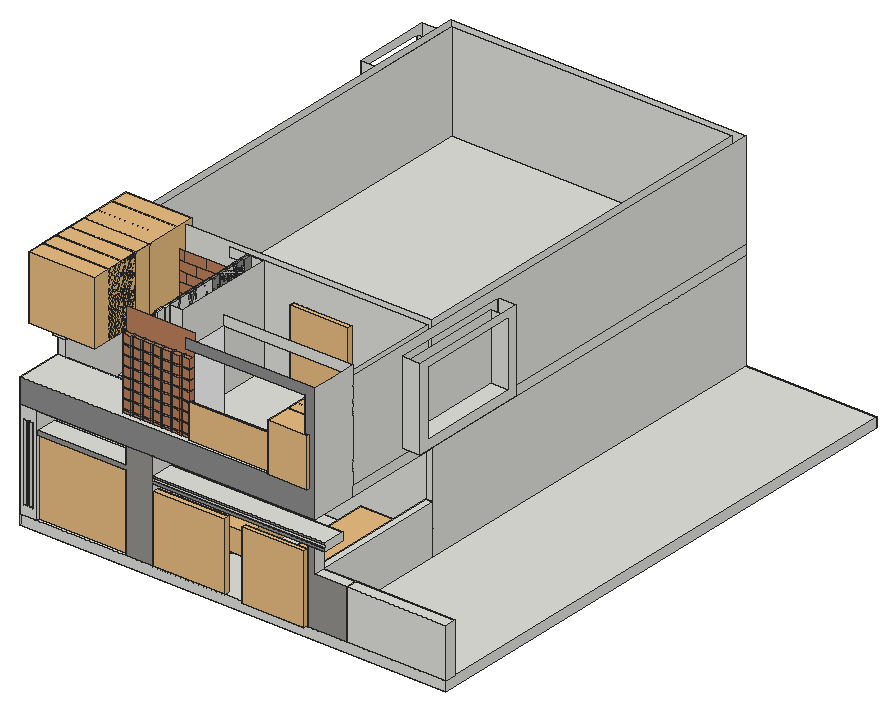
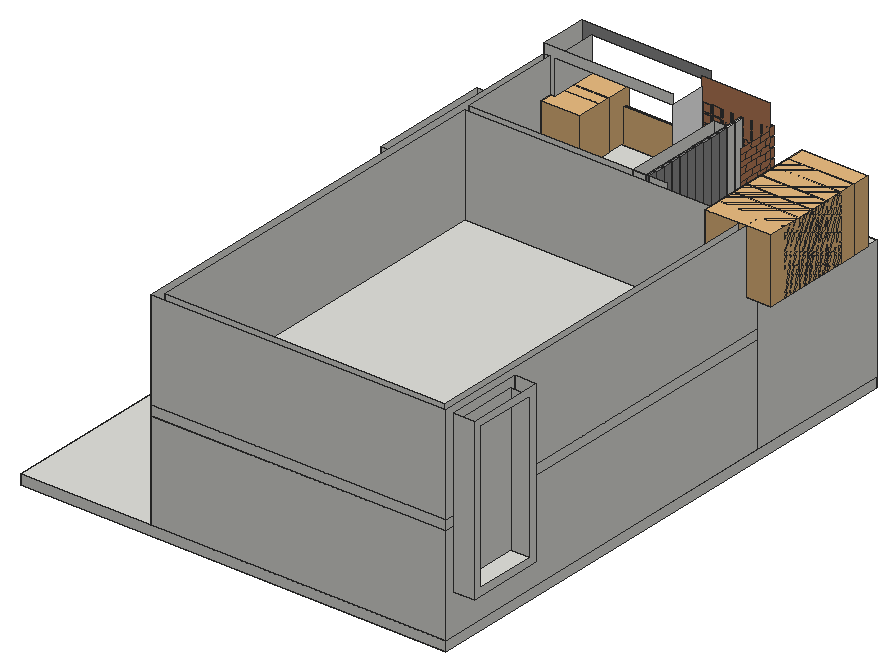
# SketchUp Ruby script. Lengths in inches.
U = 1.inch
M = Sketchup.active_model
def pt(a) = Geom::Point3d.new(a.map { |v| v * U })
def face(e, loops, mat)
  f = e.add_face(loops[0].map { |a| pt(a) })
  loops[1..].each { |l| e.add_face(l.map { |a| pt(a) }).erase! }
  f.material = f.back_material = mat if mat
  f
end
# faces: each face lists its corners as indices into pts; further lists are holes
def faces(e, pts, list, mat = nil) = list.each { |f| face(e, (f[0].is_a?(Array) ? f : [f]).map { |l| l.map { |i| pts[i] } }, mat) }
# xy, xz, yz: faces in a plane at the given z, y or x. An outline is a flat list of corners, or four numbers for a rectangle; further outlines are holes
def ring(l) = l.size == 4 ? [[l[0], l[1]], [l[2], l[1]], [l[2], l[3]], [l[0], l[3]]] : l.each_slice(2).to_a
def flat(e, list, mat, &to3) = list.each { |f| face(e, (f[0].is_a?(Array) ? f : [f]).map { |l| ring(l).map { |u, v| to3.(u, v) } }, mat) }
def xy(e, z, list, mat = nil) = flat(e, list, mat) { |x, y| [x, y, z] }
def xz(e, y, list, mat = nil) = flat(e, list, mat) { |x, z| [x, y, z] }
def yz(e, x, list, mat = nil) = flat(e, list, mat) { |y, z| [x, y, z] }
def lines(e, pts, list) = list.each { |a, b| e.add_line(pt(pts[a]), pt(pts[b])) }
# prism: a flat outline (further loops are holes) pulled along v
def prism(e, loops, v, mat = nil)
  f = face(e, loops, mat); d = Geom::Vector3d.new(v.map { |x| x * U })
  f.pushpull(f.normal.samedirection?(d) ? d.length : -d.length)
end
def box(e, o, s, mat = nil) = prism(e, [[o, [o[0] + s[0], o[1], o[2]], [o[0] + s[0], o[1] + s[1], o[2]], [o[0], o[1] + s[1], o[2]]]], [0, 0, s[2]], mat)
def at(x, y, z, deg = 0) = Geom::Transformation.translation(pt([x, y, z])) * Geom::Transformation.rotation(ORIGIN, Z_AXIS, deg.degrees)
def axes(o, x, y, z) = Geom::Transformation.new([*x, 0, *y, 0, *z, 0, *pt(o).to_a, 1])
def part(name) = M.definitions.add(name)
# library, detail: a bought-in or finely detailed component or shape, given as its bounding box
def library(name, o, s) = part(name).tap { |d| box(d.entities, o, s) }
def detail(e, o, s) = box(e.add_group.entities, o, s)
def put(e, d, t, mat = nil) = e.add_instance(d, t).tap { |i| i.material = mat if mat }
def group(e, t, mat = nil) = e.add_group.tap { |g| g.transformation = t; g.material = mat if mat }.entities
root = M.entities
M.materials.add("[Color M00]").color = [255, 255, 255]
M.materials.add("[Color M04]").color = [142, 142, 142]
M.materials.add("[Granite Light Gray]").color = [149, 148, 144]
M.materials.add("[Wood Veneer 02]").color = [190, 128, 91]
c1 = library("Untitled",[-140.43,-165.12,-406.46],[82.02,2.41,46.46])
c2 = library("Double metal gate",[0,0,0],[87.31,5.6,111.9])
c3 = library("mercy",[0,0.0625,0.17],[86.93,197.26,61.05])
c4 = library("skp127A",[-867.34,-144.26,-31.81],[70.33,146.61,36.4])
c5 = library("ske10",[-0.02,0,-0.02],[0.61,0.21,0.61])
c6 = part("Group\#44")
put(c6.entities,c5,axes([0,3814.77,792.79],[0,-1379.55262,0],[1876.19156,0,0],[0,0,-1379.55262]))
put(c6.entities,c5,axes([8.16,779.46,780.08],[0,-1356.35677,0],[1356.35677,0,0],[0,0,-1356.35677]))
c7 = part("ske69")
put(c7.entities,c4,axes([28413.25,5172.05,1237.79],[36.65,0,0],[0,36.65,0],[0,0,36.65]))
put(c7.entities,c6,at(-3177.4,833.5,-0.89))
put(c7.entities,c6,axes([-1005.07,821.63,0],[-1,0,0],[0,1,0],[0,0,1]))
c8 = part("Untitled\#1")
put(c8.entities,c7,axes([477.34,-958.1,-17.4375],[0.1036,0,0],[0,0.1036,0],[0,0,0.1036]))
c9 = part("Group\#156")
prism(c9.entities,[[[0,0,0],[0,10.0625,0],[0,10.0625,0.9],[0,10.0625,12],[0,10.0625,12.9],[0,10.0625,24.9],[0,10.0625,36.9],[0,10.0625,48.9],[0,10.0625,60.9],[0,10.0625,72.9],[0,10.0625,84.9],[0,10.0625,96.9],[0,10.0625,108.9],[0,10.0625,120.9],[0,10.0625,131.875],[0,0,131.875]]],[-3.5625,0,0])
c10 = part("Group\#155")
box(c10.entities,[0,0,0],[10,10,5.4375],"[Color M00]")
c11 = library("glass door",[0,0,0],[6.2,71.19,86.61])
c12 = library("Wagner Glass Railing",[9.08,102.375,1.53],[2.51,145.5,42.05])
c13 = library("KentiaPalm",[-22.86,-14.31,0],[47.49,43.96,59.125])
c14 = library("Round Planter with Plant",[-35.48,-39.77,0],[80.62,63.55,77.875])
xy(root,0,[[34.0625,4.36,54.1875,61.36],[162.77,4.36,196.52,30.99],[385.0625,4.43,385.0625,61.36,394.0625,61.36,394.0625,17.84,433,17.84,433,4.43],[433,4.43,554.0625,17.84],[34.0625,61.36,44.1875,184.55],
  [[44.1875,61.36,185.125,61.36,185.125,184.55,394.0625,184.55,394.0625,661.36,34.0625,661.36,34.0625,184.55,44.1875,184.55],[43.0625,193.55,385.0625,652.36]],[185.125,61.36,385.0625,70.36],[185.125,70.36,385.0625,184.55],[43.0625,193.55,385.0625,652.36]])
xy(root,11.32,[[45.66,4.36,49.72,7.36]])
xy(root,11.5,[[38.65,4.36,42.71,7.36]])
xy(root,12,[[44.1875,61.36,171.15,68.43]])
xy(root,24,[[44.1875,68.43,171.15,80.43]])
xy(root,36,[[44.1875,80.43,171.15,92.43]])
xy(root,48,[[44.1875,92.43,171.15,104.43]])
xy(root,49.1875,[[7.8125,556.61,34.0625,650.86]])
xy(root,58.14,[[7.8125,565.56,31.8125,641.91]])
xy(root,60,[[44.1875,104.43,171.15,116.43]])
xy(root,60.375,[[394.0625,4.43,433,17.84],[433,4.43,554.0625,17.84],[385.0625,17.84,394.0625,184.55]])
xy(root,72,[[44.1875,116.43,171.15,128.43]])
xy(root,84,[[44.1875,128.43,171.15,140.43]])
xy(root,89.1875,[[385.0625,4.43,394.0625,17.84]])
xy(root,89.38,[[196.52,4.36,406.2,30.99]])
xy(root,92.78,[[196.33,4.36,406.2,5.86]])
xy(root,93.625,[[54.14,4.36,162.77,30.99]])
xy(root,96,[[44.1875,140.43,171.15,152.43]])
xy(root,96.47,[[196.33,4.36,406.2,5.86]])
xy(root,98.53,[[54.14,4.36,162.77,30.99]])
xy(root,99.1875,[[196.52,4.36,406.2,30.99]])
xy(root,105.3125,[[38.65,4.36,42.71,7.36]])
xy(root,105.57,[[45.66,4.36,49.72,7.36]])
xy(root,108,[[44.1875,152.43,171.15,164.43]])
xy(root,120,[[54.1875,4.36,54.1875,61.36,394.0625,61.36,394.0625,4.36,196.52,4.36,196.52,30.99,162.77,30.99,162.77,4.36],[171.15,61.36,185.125,184.55],[185.125,61.36,394.0625,184.55],[44.1875,164.43,171.15,184.55],[[34.0625,184.55,394.0625,661.36],[43.0625,193.55,385.0625,652.36]]])
xy(root,132,[[187.02,61.36,394.0625,61.36,394.0625,61.62,387.09,61.62,387.09,184.55,187.02,184.55],[387.09,61.62,394.0625,184.55],[43.0625,193.55,385.0625,652.36]])
xy(root,140.375,[[394.0625,137.15,416.125,283.4]])
xy(root,150.125,[[34.0625,4.36,381.58,4.36,381.58,61.36,236.46,61.36,236.46,17.17,153.47,17.17,153.47,61.36,34.0625,61.36],[153.47,17.17,171.15,61.36],[171.15,17.17,236.46,61.36]])
xy(root,151.78,[[394.0625,149.62,416.125,272.62]])
xy(root,171.9375,[[31.4375,56.86,31.4375,184.55,34.0625,184.55,34.0625,61.36,44.1875,61.36,44.1875,184.55,47.125,184.55,47.125,56.86],[34.0625,61.36,44.1875,184.55]])
xy(root,175.625,[[31.4375,56.86,47.125,184.55]])
xz(root,4.36,[[[34.0625,0,54.1875,0,54.1875,93.625,54.14,93.625,54.14,98.53,54.1875,98.53,54.1875,120,34.0625,120],[45.66,11.32,49.72,105.57],[38.65,11.5,42.71,105.3125]],[54.14,93.625,54.1875,98.53]])
xz(root,4.36,[[34.0625,120,394.0625,120,394.0625,264,236.46,264,236.46,252,381.58,252,381.58,150.125,34.0625,150.125]],"[Color M04]")
xz(root,4.36,[[162.77,0,196.52,0,196.52,89.38,406.2,89.38,406.2,92.78,196.33,92.78,196.33,96.47,406.2,96.47,406.2,99.1875,196.52,99.1875,196.52,120,162.77,120,162.77,98.53,54.1875,98.53,54.1875,93.625,162.77,93.625]],"[Granite Light Gray]")
xz(root,4.43,[[433,0,554.0625,60.375]])
xz(root,4.43,[[385.0625,0,433,0,433,60.375,394.0625,60.375,394.0625,89.1875,385.0625,89.1875]],"[Granite Light Gray]")
xz(root,5.86,[[196.33,92.78,406.2,96.47]])
xz(root,7.36,[[45.66,11.32,49.72,105.57],[38.65,11.5,42.71,105.3125]])
xz(root,17.17,[[153.47,150.125,236.46,264]],"[Wood Veneer 02]")
xz(root,17.84,[[394.0625,0,433,60.375],[433,0,554.0625,60.375],[385.0625,60.375,394.0625,89.1875]])
xz(root,30.99,[[162.77,0,162.77,93.625,54.14,93.625,54.14,98.53,162.77,98.53,162.77,120,196.52,120,196.52,99.1875,406.2,99.1875,406.2,89.38,196.52,89.38,196.52,0]])
xz(root,56.86,[[31.4375,171.9375,47.125,175.625]])
xz(root,61.36,[[44.1875,0,54.1875,12],[54.1875,0,185.125,0,185.125,120,171.15,120,171.15,12,54.1875,12],[44.1875,120,171.15,132],[171.15,120,305.4,132],[305.4,120,394.0625,132],
  [44.1875,132,171.15,150.125],[171.15,132,187.02,150.125],[187.02,132,187.02,150.125,381.58,150.125,381.58,252,236.46,252,236.46,264,394.0625,264,394.0625,132],[34.0625,150.125,44.1875,171.9375],[171.15,150.125,187.02,251.875]])
xz(root,61.62,[[387.09,132,394.0625,252]])
xz(root,68.43,[[44.1875,12,171.15,24]])
xz(root,80.43,[[44.1875,24,171.15,36]])
xz(root,92.43,[[44.1875,36,171.15,48]])
xz(root,104.43,[[44.1875,48,171.15,60]])
xz(root,116.43,[[44.1875,60,171.15,72]])
xz(root,128.43,[[44.1875,72,171.15,84]])
xz(root,137.15,[[394.0625,140.375,416.125,240.5]])
xz(root,140.43,[[44.1875,84,171.15,96]])
xz(root,149.62,[[394.0625,151.78,416.125,231.53]])
xz(root,152.43,[[44.1875,96,171.15,108]])
xz(root,164.43,[[44.1875,108,171.15,120]])
xz(root,184.55,[[34.0625,0,44.1875,120],[185.125,0,385.0625,120],[385.0625,0,394.0625,60.375],[385.0625,60.375,394.0625,120],[171.15,120,394.0625,132],
  [34.0625,132,43.0625,171.9375],[43.0625,132,44.1875,132.9],[187.02,132,387.09,132,387.09,252,145.79,252,145.79,240.9,171.15,240.9,171.15,251.875,187.02,251.875],[171.15,132,187.02,251.875],[43.0625,132.9,44.1875,144.9],
  [43.0625,144.9,44.1875,156.9],[43.0625,156.9,44.1875,168.9],[43.0625,168.9,44.1875,171.9375],[31.4375,171.9375,34.0625,175.625],[34.0625,171.9375,43.0625,175.625],
  [43.0625,171.9375,47.125,175.625],[34.0625,175.625,43.0625,252]])
xz(root,184.55,[[34.0625,120,44.1875,132],[44.1875,120,67.86,120.9],[67.86,120,171.15,120.9]],"[Color M00]")
xz(root,184.55,[[44.1875,120.9,67.86,132.9],[67.86,120.9,92.41,132.9],[92.41,120.9,118.04,132.9],[118.04,120.9,142.75,132.9],[142.75,120.9,162.77,132.9],
  [162.77,120.9,171.15,132.9],[44.1875,132.9,55.875,144.9],[55.875,132.9,79.83,144.9],[79.83,132.9,104.98,144.9],[104.98,132.9,131.1,144.9],
  [131.1,132.9,154.39,144.9],[154.39,132.9,171.15,144.9],[44.1875,144.9,67.57,156.9],[67.57,144.9,92.1,156.9],[92.1,144.9,117.85,156.9],
  [117.85,144.9,144.35,156.9],[144.35,144.9,164.4375,156.9],[164.4375,144.9,171.15,156.9],[44.1875,156.9,55.66,168.9],[55.66,156.9,79.47,168.9],
  [79.47,156.9,104.73,168.9],[104.73,156.9,130.97,168.9],[130.97,156.9,157.73,168.9],[157.73,156.9,171.15,168.9],[44.1875,168.9,67.125,168.9,67.125,180.9,43.0625,180.9,43.0625,175.625,47.125,175.625,47.125,171.9375,44.1875,171.9375],
  [67.125,168.9,91.82,180.9],[91.82,168.9,117.64,180.9],[117.64,168.9,144.3,180.9],[144.3,168.9,171.15,180.9],[43.0625,180.9,55.02,192.9],
  [55.02,180.9,79.23,192.9],[79.23,180.9,104.42,192.9],[104.42,180.9,130.85,192.9],[130.85,180.9,157.74,192.9],[157.74,180.9,171.15,192.9],
  [43.0625,192.9,66.98,204.9],[66.98,192.9,91.47,204.9],[91.47,192.9,117.38,204.9],[117.38,192.9,144.33,204.9],[144.33,192.9,171.15,204.9],
  [43.0625,204.9,55,216.9],[55,204.9,78.96,216.9],[78.96,204.9,103.97,216.9],[103.97,204.9,130.78,216.9],[130.78,204.9,157.88,216.9],
  [157.88,204.9,171.15,216.9],[43.0625,216.9,66.9375,228.9],[66.9375,216.9,90.99,228.9],[90.99,216.9,116.95,228.9],[116.95,216.9,144.61,228.9],
  [144.61,216.9,171.15,228.9]],"[Wood Veneer 02]")
xz(root,193.55,[[43.0625,0,385.0625,120],[43.0625,132,385.0625,252]])
xz(root,272.62,[[394.0625,151.78,416.125,231.53]])
xz(root,283.4,[[394.0625,140.375,416.125,240.5]])
xz(root,556.61,[[7.8125,49.1875,34.0625,244.31]])
xz(root,565.56,[[7.8125,58.14,31.8125,235.36]])
xz(root,641.91,[[7.8125,58.14,31.8125,235.36]])
xz(root,650.86,[[7.8125,49.1875,34.0625,244.31]])
xz(root,652.36,[[43.0625,0,385.0625,120],[43.0625,132,385.0625,252]])
xz(root,661.36,[[34.0625,0,394.0625,120],[34.0625,120,394.0625,132],[34.0625,132,394.0625,252]])
yz(root,7.8125,[[[556.61,49.1875,650.86,244.31],[565.56,58.14,641.91,235.36]]])
yz(root,31.4375,[[56.86,171.9375,184.55,175.625]])
yz(root,31.8125,[[565.56,58.14,641.91,235.36]])
yz(root,34.0625,[[4.36,0,4.36,150.125,61.36,150.125,61.36,171.9375,184.55,171.9375,184.55,0],[184.55,0,184.55,120,556.61,120,556.61,49.1875,650.86,49.1875,650.86,120,661.36,120,661.36,0],[556.61,49.1875,650.86,120],[184.55,120,556.61,132],[650.86,120,661.36,132],
  [184.55,132,184.55,252,661.36,252,661.36,132,650.86,132,650.86,244.31,556.61,244.31,556.61,132]])
yz(root,38.65,[[4.36,11.5,7.36,105.3125]])
yz(root,42.71,[[4.36,11.5,7.36,105.3125]])
yz(root,43.0625,[[193.55,0,652.36,120],[193.55,132,652.36,252]])
yz(root,44.1875,[[61.36,12,68.43,12,68.43,24,80.43,24,80.43,36,92.43,36,92.43,48,104.43,48,104.43,60,116.43,60,116.43,72,128.43,72,128.43,84,140.43,84,140.43,96,152.43,96,152.43,108,164.43,108,164.43,171.9375,61.36,171.9375],[164.43,120,184.55,171.9375]])
yz(root,45.66,[[4.36,11.32,7.36,105.57]])
yz(root,47.125,[[56.86,171.9375,184.55,175.625]])
yz(root,49.72,[[4.36,11.32,7.36,105.57]])
yz(root,54.14,[[4.36,93.625,30.99,98.53]])
yz(root,54.1875,[[4.36,0,61.36,120]])
yz(root,153.47,[[17.17,150.125,24.05,159.72],[24.05,150.125,38.34,159.72],[38.34,150.125,53.5625,159.72],[53.5625,150.125,61.36,159.72],[17.17,159.72,30.92,168.68],
  [30.92,159.72,45.76,168.68],[45.76,159.72,61.36,168.68],[17.17,168.68,23.81,177.77],[23.81,168.68,38.03,177.77],[38.03,168.68,53.49,177.77],
  [53.49,168.68,61.36,177.77],[17.17,177.77,30.4375,186.99],[30.4375,177.77,45.625,186.99],[45.625,177.77,61.36,186.99],[17.17,186.99,22.72,195.85],
  [22.72,186.99,38.15,195.85],[38.15,186.99,53.09,195.85],[53.09,186.99,61.36,195.85],[17.17,195.85,31.48,203.71],[31.48,195.85,44.83,203.71],
  [44.83,195.85,61.36,203.71],[17.17,203.71,24.23,211.55],[24.23,203.71,38.73,211.55],[38.73,203.71,53.77,211.55],[53.77,203.71,61.36,211.55],
  [17.17,211.55,31.29,218.4375],[31.29,211.55,46.18,218.4375],[46.18,211.55,61.36,218.4375],[17.17,218.4375,24.45,225.95],[24.45,218.4375,38.13,225.95],
  [38.13,218.4375,54.23,225.95],[54.23,218.4375,61.36,225.95],[17.17,225.95,31.72,233.2],[31.72,225.95,47.09,233.2],[47.09,225.95,61.36,233.2]],"[Wood Veneer 02]")
yz(root,162.77,[[4.36,0,30.99,93.625],[4.36,98.53,30.99,120]])
yz(root,171.15,[[61.36,12,61.36,120,164.43,120,164.43,108,152.43,108,152.43,96,140.43,96,140.43,84,128.43,84,128.43,72,116.43,72,116.43,60,104.43,60,104.43,48,92.43,48,92.43,36,80.43,36,80.43,24,68.43,24,68.43,12],[61.36,120,174.49,251.875]])
yz(root,185.125,[[61.36,0,184.55,120]])
yz(root,187.02,[[61.36,132,184.55,251.875]])
yz(root,196.33,[[4.36,92.78,5.86,96.47]])
yz(root,196.52,[[4.36,0,30.99,89.38],[4.36,99.1875,30.99,120]])
yz(root,236.46,[[17.17,150.125,61.36,252]],"[Color M00]")
yz(root,381.58,[[4.36,150.125,61.36,252]])
yz(root,385.0625,[[4.43,0,4.43,89.1875,17.84,89.1875,17.84,60.375,70.36,60.375,70.36,0],[70.36,0,184.55,60.375],[193.55,0,652.36,120],[193.55,132,652.36,252]])
yz(root,387.09,[[61.62,132,184.55,252]])
yz(root,394.0625,[[17.84,0,184.55,60.375],[184.55,0,661.36,120],[4.43,60.375,17.84,89.1875],[4.36,120,61.36,120,61.36,264,27.86,263.93,27.86,264,4.36,264],[61.36,120,184.55,132],
  [184.55,120,661.36,132],[[61.62,132,661.36,252],[137.15,140.375,283.4,240.5]],[149.62,151.78,272.62,231.53]])
yz(root,406.2,[[4.36,89.38,30.99,89.38,30.99,99.1875,4.36,99.1875,4.36,96.47,5.86,96.47,5.86,92.78,4.36,92.78]])
yz(root,416.125,[[[137.15,140.375,283.4,240.5],[149.62,151.78,272.62,231.53]]])
yz(root,433,[[4.43,0,17.84,60.375]])
yz(root,554.0625,[[4.43,0,17.84,60.375]])
p = [[44.1875,61.36,132],[34.0625,61.36,132],[43.0625,184.55,120.9],[44.1875,184.55,120.9],[43.0625,184.55,108.9],[44.1875,184.55,108.9],
  [171.15,184.55,108.9],[43.0625,184.55,96.9],[44.1875,184.55,96.9],[171.15,184.55,96.9],[43.0625,184.55,84.9],[44.1875,184.55,84.9],
  [171.15,184.55,84.9],[43.0625,184.55,72.9],[44.1875,184.55,72.9],[171.15,184.55,72.9],[43.0625,184.55,60.9],[44.1875,184.55,60.9],
  [171.15,184.55,60.9],[43.0625,184.55,48.9],[44.1875,184.55,48.9],[171.15,184.55,48.9],[43.0625,184.55,36.9],[44.1875,184.55,36.9],
  [171.15,184.55,36.9],[43.0625,184.55,24.9],[44.1875,184.55,24.9],[171.15,184.55,24.9],[43.0625,184.55,12.9],[44.1875,184.55,12.9],
  [171.15,184.55,12.9],[43.0625,184.55,0.9],[44.1875,184.55,0.9],[171.15,184.55,0.9],[44.1875,61.36,120],[34.0625,61.36,120]]
lines(root,p,[[0,1],[2,3],[4,5],[5,6],[7,8],[8,9],[10,11],[11,12],[13,14],[14,15],[16,17],[17,18],
  [19,20],[20,21],[22,23],[23,24],[25,26],[26,27],[28,29],[29,30],[31,32],[32,33],[34,35]])
g1 = group(root,at(34.0625,661.36,-12))
box(g1,[0,-657,0],[520,657,12])
put(root,c1,axes([241.03,173.28,840.82],[1.33986,0,0],[0,1,0],[0,0,2.07692]))
put(root,c2,axes([196.52,4.36,-0.64],[1,0,0],[0,1,0],[0,0,0.7452]))
put(root,c3,axes([359.07,174.68,-0.375],[-0.5254,0,0],[0,-0.5254,0],[0,0,0.5254]))
put(root,c2,axes([308,0,0.61],[0.87,0,0],[0,1,0],[0,0,0.7452]))
put(root,c8,axes([186.21,255.39,6.7],[0.1953,0,0],[0,0.1953,0],[0,0,0.1953]))
put(root,c9,at(171.15,42.49,120))
put(root,c9,at(171.15,54.49,120))
put(root,c9,at(171.15,66.49,120),"[Color M04]")
put(root,c9,at(171.15,78.49,120),"[Color M04]")
put(root,c9,at(171.15,90.49,120),"[Color M04]")
put(root,c9,at(171.15,102.49,120),"[Color M04]")
put(root,c9,at(171.15,114.49,120),"[Color M04]")
put(root,c9,at(171.15,126.49,120),"[Color M04]")
put(root,c9,at(171.15,138.49,120),"[Color M04]")
put(root,c9,at(171.15,150.49,120),"[Color M04]")
put(root,c9,at(171.15,162.49,120),"[Color M04]")
put(root,c9,at(171.15,174.49,120),"[Color M04]")
put(root,c10,axes([153.47,17.17,130.41],[1,0,0],[0,0,1],[0,-1,0]))
put(root,c10,axes([189.47,17.17,130.41],[1,0,0],[0,0,1],[0,-1,0]))
put(root,c10,axes([213.47,17.17,130.41],[1,0,0],[0,0,1],[0,-1,0]))
put(root,c10,axes([201.47,17.17,130.41],[1,0,0],[0,0,1],[0,-1,0]))
put(root,c10,axes([165.47,17.17,130.41],[1,0,0],[0,0,1],[0,-1,0]))
put(root,c10,axes([177.47,17.17,130.41],[1,0,0],[0,0,1],[0,-1,0]))
put(root,c10,axes([225.47,17.17,130.41],[1,0,0],[0,0,1],[0,-1,0]))
put(root,c11,at(223.74,184.55,132,-90))
g2 = group(root,at(153.47,17.17,142.41))
box(g2,[0,-5.4375,0],[10,5.4375,10],"[Wood Veneer 02]")
g3 = group(root,at(189.47,17.17,142.41))
box(g3,[0,-5.4375,0],[10,5.4375,10],"[Wood Veneer 02]")
g4 = group(root,at(213.47,17.17,142.41))
box(g4,[0,-5.4375,0],[10,5.4375,10],"[Wood Veneer 02]")
g5 = group(root,at(201.47,17.17,142.41))
box(g5,[0,-5.4375,0],[10,5.4375,10],"[Wood Veneer 02]")
g6 = group(root,at(165.47,17.17,142.41))
box(g6,[0,-5.4375,0],[10,5.4375,10],"[Wood Veneer 02]")
g7 = group(root,at(177.47,17.17,142.41))
box(g7,[0,-5.4375,0],[10,5.4375,10],"[Wood Veneer 02]")
g8 = group(root,at(225.47,17.17,142.41))
box(g8,[0,-5.4375,0],[10,5.4375,10],"[Wood Veneer 02]")
put(root,c12,at(134.06,19.89,148.61,-90))
put(root,c13,at(361.23,46.96,151.3))
put(root,c13,at(361.23,16.15,151.3))
g9 = group(root,at(153.47,17.17,154.41),"[Wood Veneer 02]")
box(g9,[0,-5.4375,0],[10,5.4375,10],"[Wood Veneer 02]")
g10 = group(root,at(189.47,17.17,154.41))
box(g10,[0,-5.4375,0],[10,5.4375,10],"[Wood Veneer 02]")
g11 = group(root,at(213.47,17.17,154.41))
box(g11,[0,-5.4375,0],[10,5.4375,10],"[Wood Veneer 02]")
g12 = group(root,at(201.47,17.17,154.41))
box(g12,[0,-5.4375,0],[10,5.4375,10],"[Wood Veneer 02]")
g13 = group(root,at(165.47,17.17,154.41))
box(g13,[0,-5.4375,0],[10,5.4375,10],"[Wood Veneer 02]")
g14 = group(root,at(177.47,17.17,154.41))
box(g14,[0,-5.4375,0],[10,5.4375,10],"[Wood Veneer 02]")
g15 = group(root,at(225.47,17.17,154.41))
box(g15,[0,-5.4375,0],[10,5.4375,10],"[Wood Veneer 02]")
g16 = group(root,at(153.47,17.17,166.41))
box(g16,[0,-5.4375,0],[10,5.4375,10],"[Wood Veneer 02]")
g17 = group(root,at(189.47,17.17,166.41))
box(g17,[0,-5.4375,0],[10,5.4375,10],"[Wood Veneer 02]")
g18 = group(root,at(213.47,17.17,166.41))
box(g18,[0,-5.4375,0],[10,5.4375,10],"[Wood Veneer 02]")
g19 = group(root,at(201.47,17.17,166.41))
box(g19,[0,-5.4375,0],[10,5.4375,10],"[Wood Veneer 02]")
g20 = group(root,at(165.47,17.17,166.41))
box(g20,[0,-5.4375,0],[10,5.4375,10],"[Wood Veneer 02]")
g21 = group(root,at(177.47,17.17,166.41))
box(g21,[0,-5.4375,0],[10,5.4375,10],"[Wood Veneer 02]")
g22 = group(root,at(225.47,17.17,166.41))
box(g22,[0,-5.4375,0],[10,5.4375,10],"[Wood Veneer 02]")
put(root,c14,at(38.71,180.33,175.625))
put(root,c14,at(38.71,158.14,175.625))
put(root,c14,at(38.71,136.51,175.625))
put(root,c14,at(38.71,116.7,175.625))
put(root,c14,at(38.71,94.95,175.625))
g23 = group(root,at(153.47,17.17,178.41))
box(g23,[0,-5.4375,0],[10,5.4375,10],"[Wood Veneer 02]")
g24 = group(root,at(189.47,17.17,178.41))
box(g24,[0,-5.4375,0],[10,5.4375,10],"[Wood Veneer 02]")
g25 = group(root,at(213.47,17.17,178.41))
box(g25,[0,-5.4375,0],[10,5.4375,10],"[Wood Veneer 02]")
g26 = group(root,at(201.47,17.17,178.41))
box(g26,[0,-5.4375,0],[10,5.4375,10],"[Wood Veneer 02]")
g27 = group(root,at(165.47,17.17,178.41))
box(g27,[0,-5.4375,0],[10,5.4375,10],"[Wood Veneer 02]")
g28 = group(root,at(177.47,17.17,178.41))
box(g28,[0,-5.4375,0],[10,5.4375,10],"[Wood Veneer 02]")
g29 = group(root,at(225.47,17.17,178.41))
box(g29,[0,-5.4375,0],[10,5.4375,10],"[Wood Veneer 02]")
g30 = group(root,at(153.47,17.17,190.41))
box(g30,[0,-5.4375,0],[10,5.4375,10],"[Wood Veneer 02]")
g31 = group(root,at(189.47,17.17,190.41))
box(g31,[0,-5.4375,0],[10,5.4375,10],"[Wood Veneer 02]")
g32 = group(root,at(213.47,17.17,190.41))
box(g32,[0,-5.4375,0],[10,5.4375,10],"[Wood Veneer 02]")
g33 = group(root,at(201.47,17.17,190.41))
box(g33,[0,-5.4375,0],[10,5.4375,10],"[Wood Veneer 02]")
g34 = group(root,at(165.47,17.17,190.41))
box(g34,[0,-5.4375,0],[10,5.4375,10],"[Wood Veneer 02]")
g35 = group(root,at(177.47,17.17,190.41))
box(g35,[0,-5.4375,0],[10,5.4375,10],"[Wood Veneer 02]")
g36 = group(root,at(225.47,17.17,190.41))
box(g36,[0,-5.4375,0],[10,5.4375,10],"[Wood Veneer 02]")
g37 = group(root,at(153.47,17.17,202.41))
box(g37,[0,-5.4375,0],[10,5.4375,10],"[Wood Veneer 02]")
g38 = group(root,at(189.47,17.17,202.41))
box(g38,[0,-5.4375,0],[10,5.4375,10],"[Wood Veneer 02]")
g39 = group(root,at(213.47,17.17,202.41))
box(g39,[0,-5.4375,0],[10,5.4375,10],"[Wood Veneer 02]")
g40 = group(root,at(201.47,17.17,202.41))
box(g40,[0,-5.4375,0],[10,5.4375,10],"[Wood Veneer 02]")
g41 = group(root,at(165.47,17.17,202.41))
box(g41,[0,-5.4375,0],[10,5.4375,10],"[Wood Veneer 02]")
g42 = group(root,at(177.47,17.17,202.41))
box(g42,[0,-5.4375,0],[10,5.4375,10],"[Wood Veneer 02]")
g43 = group(root,at(225.47,17.17,202.41))
box(g43,[0,-5.4375,0],[10,5.4375,10],"[Wood Veneer 02]")
g44 = group(root,at(189.47,17.17,214.41))
box(g44,[0,-5.4375,0],[10,5.4375,10],"[Wood Veneer 02]")
g45 = group(root,at(153.47,17.17,214.41))
box(g45,[0,-5.4375,0],[10,5.4375,10],"[Wood Veneer 02]")
g46 = group(root,at(213.47,17.17,214.41))
box(g46,[0,-5.4375,0],[10,5.4375,10],"[Wood Veneer 02]")
g47 = group(root,at(201.47,17.17,214.41))
box(g47,[0,-5.4375,0],[10,5.4375,10],"[Wood Veneer 02]")
g48 = group(root,at(165.47,17.17,214.41))
box(g48,[0,-5.4375,0],[10,5.4375,10],"[Wood Veneer 02]")
g49 = group(root,at(177.47,17.17,214.41))
box(g49,[0,-5.4375,0],[10,5.4375,10],"[Wood Veneer 02]")
g50 = group(root,at(225.47,17.17,214.41))
box(g50,[0,-5.4375,0],[10,5.4375,10],"[Wood Veneer 02]")
g51 = group(root,at(153.47,17.17,226.41))
box(g51,[0,-5.4375,0],[10,5.4375,10],"[Wood Veneer 02]")
g52 = group(root,at(189.47,17.17,226.41))
box(g52,[0,-5.4375,0],[10,5.4375,10],"[Wood Veneer 02]")
g53 = group(root,at(213.47,17.17,226.41))
box(g53,[0,-5.4375,0],[10,5.4375,10],"[Wood Veneer 02]")
g54 = group(root,at(201.47,17.17,226.41))
box(g54,[0,-5.4375,0],[10,5.4375,10],"[Wood Veneer 02]")
g55 = group(root,at(165.47,17.17,226.41))
box(g55,[0,-5.4375,0],[10,5.4375,10],"[Wood Veneer 02]")
g56 = group(root,at(177.47,17.17,226.41))
box(g56,[0,-5.4375,0],[10,5.4375,10],"[Wood Veneer 02]")
g57 = group(root,at(225.47,17.17,226.41))
box(g57,[0,-5.4375,0],[10,5.4375,10],"[Wood Veneer 02]")
